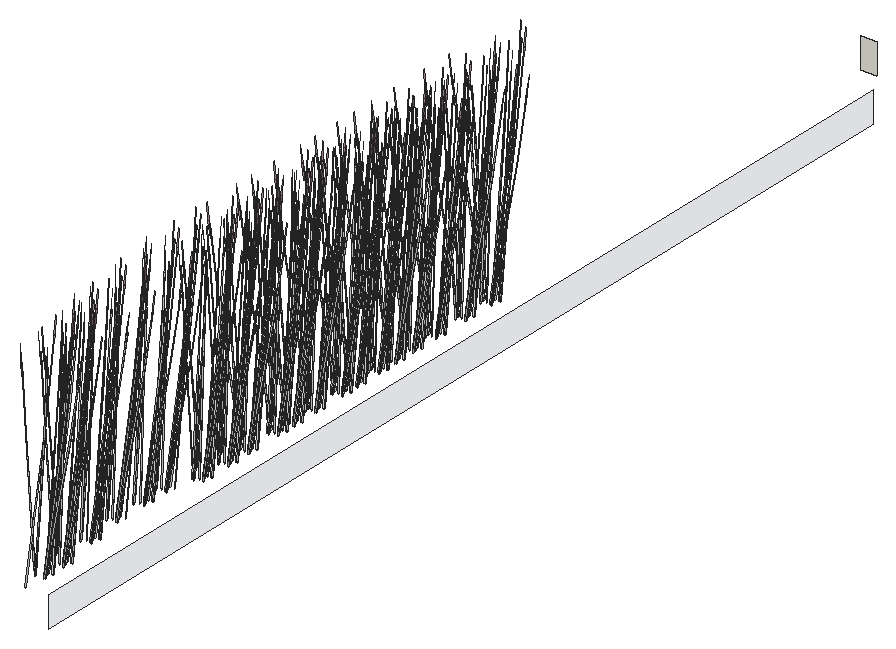
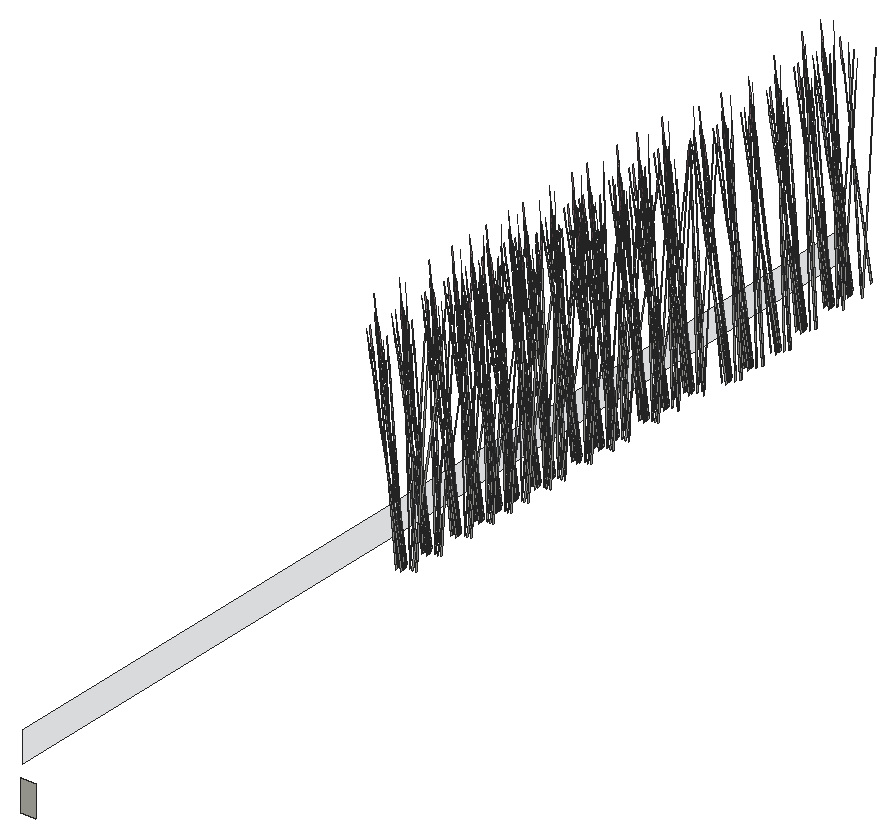
# SketchUp Ruby script. Lengths in inches.
U = 1.inch
M = Sketchup.active_model
def pt(a) = Geom::Point3d.new(a.map { |v| v * U })
def face(e, loops, mat)
  f = e.add_face(loops[0].map { |a| pt(a) })
  loops[1..].each { |l| e.add_face(l.map { |a| pt(a) }).erase! }
  f.material = f.back_material = mat if mat
  f
end
# faces: each face lists its corners as indices into pts; further lists are holes
def faces(e, pts, list, mat = nil) = list.each { |f| face(e, (f[0].is_a?(Array) ? f : [f]).map { |l| l.map { |i| pts[i] } }, mat) }
# xy, xz, yz: faces in a plane at the given z, y or x. An outline is a flat list of corners, or four numbers for a rectangle; further outlines are holes
def ring(l) = l.size == 4 ? [[l[0], l[1]], [l[2], l[1]], [l[2], l[3]], [l[0], l[3]]] : l.each_slice(2).to_a
def flat(e, list, mat, &to3) = list.each { |f| face(e, (f[0].is_a?(Array) ? f : [f]).map { |l| ring(l).map { |u, v| to3.(u, v) } }, mat) }
def xy(e, z, list, mat = nil) = flat(e, list, mat) { |x, y| [x, y, z] }
def xz(e, y, list, mat = nil) = flat(e, list, mat) { |x, z| [x, y, z] }
def yz(e, x, list, mat = nil) = flat(e, list, mat) { |y, z| [x, y, z] }
def lines(e, pts, list) = list.each { |a, b| e.add_line(pt(pts[a]), pt(pts[b])) }
# prism: a flat outline (further loops are holes) pulled along v
def prism(e, loops, v, mat = nil)
  f = face(e, loops, mat); d = Geom::Vector3d.new(v.map { |x| x * U })
  f.pushpull(f.normal.samedirection?(d) ? d.length : -d.length)
end
def box(e, o, s, mat = nil) = prism(e, [[o, [o[0] + s[0], o[1], o[2]], [o[0] + s[0], o[1] + s[1], o[2]], [o[0], o[1] + s[1], o[2]]]], [0, 0, s[2]], mat)
def at(x, y, z, deg = 0) = Geom::Transformation.translation(pt([x, y, z])) * Geom::Transformation.rotation(ORIGIN, Z_AXIS, deg.degrees)
def axes(o, x, y, z) = Geom::Transformation.new([*x, 0, *y, 0, *z, 0, *pt(o).to_a, 1])
def part(name) = M.definitions.add(name)
# library, detail: a bought-in or finely detailed component or shape, given as its bounding box
def library(name, o, s) = part(name).tap { |d| box(d.entities, o, s) }
def detail(e, o, s) = box(e.add_group.entities, o, s)
def put(e, d, t, mat = nil) = e.add_instance(d, t).tap { |i| i.material = mat if mat }
def group(e, t, mat = nil) = e.add_group.tap { |g| g.transformation = t; g.material = mat if mat }.entities
root = M.entities
M.materials.add("D01_Frost_White").color = [238, 238, 227]
M.materials.add("Glass_Basic_01").color = [161, 173, 186]
M.materials["Glass_Basic_01"].alpha = 0.25
M.materials.add("LightPink_Translucent").color = [144, 107, 117]
M.materials["LightPink_Translucent"].alpha = 0.75
c1 = part("blade")
p = [[2.15,0.21,22],[0,0.17,0],[0.09,0.45,0],[2.18,0.31,22],[2.29,0.31,22],[0.38,0.45,0],
  [2.48,0.24,33],[2.49,0.24,33],[2.48,0.22,33]]
faces(c1.entities,p,[[0,1,2,3],[4,5,2,3],[6,3,4,7],[8,0,3,6]])
c2 = part("seeds")
p = [[0.3,-0.1,1.38],[-0.01,-0.03,1.59],[-0.01,-0.03,0.03],[0.14,-0.07,-0.07],[0.29,-0.03,3],[0.15,0.01,3.11]]
faces(c2.entities,p,[[0,1,2,3],[1,0,4,5]],"LightPink_Translucent")
c3 = part("blade with seeds")
put(c3.entities,c1,at(0,0,0))
put(c3.entities,c2,axes([2.4,0.25,30.99],[1.5799,-0.05474,1.17369],[-0.12525,1.92788,0.29478],[-0.07173,-0.02425,1.56792]))
xz(root,586,[[427,150,430,156]],"D01_Frost_White")
yz(root,439,[[373,150,574.02,156]],"Glass_Basic_01")
put(root,c3,axes([428.45,433.25,151.77],[-0.1683,-0.48366,-0.58997],[0.48479,-0.17419,-0.15484],[-0.0186,-0.16378,1.30225]))
put(root,c3,axes([428.45,440.5,151.77],[-0.1683,-0.48366,-0.58997],[0.48479,-0.17419,-0.15484],[-0.0186,-0.16378,1.30225]))
put(root,c3,axes([428.45,444.2,151.77],[-0.1683,-0.48366,-0.58997],[0.48479,-0.17419,-0.15484],[-0.0186,-0.16378,1.30225]))
put(root,c3,axes([428.45,449.62,151.77],[-0.1683,-0.48366,-0.58997],[0.48479,-0.17419,-0.15484],[-0.0186,-0.16378,1.30225]))
put(root,c3,axes([428.45,456.1,151.77],[-0.1683,-0.48366,-0.58997],[0.48479,-0.17419,-0.15484],[-0.0186,-0.16378,1.30225]))
put(root,c3,axes([428.45,459.65,151.77],[-0.1683,-0.48366,-0.58997],[0.48479,-0.17419,-0.15484],[-0.0186,-0.16378,1.30225]))
put(root,c3,axes([428.45,465.05,151.77],[-0.1683,-0.48366,-0.58997],[0.48479,-0.17419,-0.15484],[-0.0186,-0.16378,1.30225]))
put(root,c3,axes([428.45,469.1,151.77],[-0.1683,-0.48366,-0.58997],[0.48479,-0.17419,-0.15484],[-0.0186,-0.16378,1.30225]))
put(root,c3,axes([428.45,473.43,151.77],[-0.1683,-0.48366,-0.58997],[0.48479,-0.17419,-0.15484],[-0.0186,-0.16378,1.30225]))
put(root,c3,axes([428.45,478.97,151.77],[-0.1683,-0.48366,-0.58997],[0.48479,-0.17419,-0.15484],[-0.0186,-0.16378,1.30225]))
put(root,c3,axes([428.45,486.18,151.77],[-0.1683,-0.48366,-0.58997],[0.48479,-0.17419,-0.15484],[-0.0186,-0.16378,1.30225]))
put(root,c3,axes([428.45,492.34,151.77],[-0.1683,-0.48366,-0.58997],[0.48479,-0.17419,-0.15484],[-0.0186,-0.16378,1.30225]))
put(root,c3,axes([427.55,404.96,151.77],[0.15027,0.43184,-0.5847],[-0.43285,0.15553,-0.15346],[0.01661,0.14623,1.29063]))
put(root,c3,axes([428.4,397.25,151.87],[-0.19883,0.425,-0.37796],[-0.41314,-0.20454,0.1819],[0,0.09797,1.2135]))
put(root,c3,axes([428.51,411.5625,151.71],[-0.28606,0.29428,-0.2617],[-0.28606,-0.29428,0.2617],[0,0.09479,1.17405]))
put(root,c3,axes([427.62,416.89,151.77],[0.15027,0.43184,-0.5847],[-0.43285,0.15553,-0.15346],[0.01661,0.14623,1.29063]))
put(root,c3,axes([427.69,411.51,151.77],[0.15027,0.43184,-0.5847],[-0.43285,0.15553,-0.15346],[0.01661,0.14623,1.29063]))
put(root,c3,axes([427.65,383.51,151.71],[0.28606,-0.29428,-0.2617],[0.28606,0.29428,0.2617],[0,-0.09479,1.17405]))
put(root,c3,axes([427.65,388.08,151.71],[0.28606,-0.29428,-0.2617],[0.28606,0.29428,0.2617],[0,-0.09479,1.17405]))
put(root,c3,axes([427.65,422.17,151.71],[0.28606,-0.29428,-0.2617],[0.28606,0.29428,0.2617],[0,-0.09479,1.17405]))
put(root,c3,axes([427.65,428.28,151.71],[0.28606,-0.29428,-0.2617],[0.28606,0.29428,0.2617],[0,-0.09479,1.17405]))
put(root,c3,axes([427.65,433.19,151.71],[0.28606,-0.29428,-0.2617],[0.28606,0.29428,0.2617],[0,-0.09479,1.17405]))
put(root,c3,axes([427.65,440.45,151.71],[0.28606,-0.29428,-0.2617],[0.28606,0.29428,0.2617],[0,-0.09479,1.17405]))
put(root,c3,axes([427.65,444.14,151.71],[0.28606,-0.29428,-0.2617],[0.28606,0.29428,0.2617],[0,-0.09479,1.17405]))
put(root,c3,axes([427.65,449.5625,151.71],[0.28606,-0.29428,-0.2617],[0.28606,0.29428,0.2617],[0,-0.09479,1.17405]))
put(root,c3,axes([427.65,456.04,151.71],[0.28606,-0.29428,-0.2617],[0.28606,0.29428,0.2617],[0,-0.09479,1.17405]))
put(root,c3,axes([427.65,459.59,151.71],[0.28606,-0.29428,-0.2617],[0.28606,0.29428,0.2617],[0,-0.09479,1.17405]))
put(root,c3,axes([427.65,464.99,151.71],[0.28606,-0.29428,-0.2617],[0.28606,0.29428,0.2617],[0,-0.09479,1.17405]))
put(root,c3,axes([427.65,469.05,151.71],[0.28606,-0.29428,-0.2617],[0.28606,0.29428,0.2617],[0,-0.09479,1.17405]))
put(root,c3,axes([427.65,473.37,151.71],[0.28606,-0.29428,-0.2617],[0.28606,0.29428,0.2617],[0,-0.09479,1.17405]))
put(root,c3,axes([427.65,478.91,151.71],[0.28606,-0.29428,-0.2617],[0.28606,0.29428,0.2617],[0,-0.09479,1.17405]))
put(root,c3,axes([427.65,486.12,151.71],[0.28606,-0.29428,-0.2617],[0.28606,0.29428,0.2617],[0,-0.09479,1.17405]))
put(root,c3,axes([427.65,492.29,151.71],[0.28606,-0.29428,-0.2617],[0.28606,0.29428,0.2617],[0,-0.09479,1.17405]))
put(root,c3,axes([426.38,402.86,151.71],[0.38233,0.1167,-0.2617],[-0.09626,0.41098,0.2617],[0.07708,-0.04739,1.17405]))
put(root,c3,axes([426.45,414.79,151.71],[0.38233,0.1167,-0.2617],[-0.09626,0.41098,0.2617],[0.07708,-0.04739,1.17405]))
put(root,c3,axes([426.52,409.41,151.71],[0.38233,0.1167,-0.2617],[-0.09626,0.41098,0.2617],[0.07708,-0.04739,1.17405]))
put(root,c3,axes([428.56,405.02,151.7],[0,0.47166,-0.41945],[-0.45849,0,0],[0,0.10742,1.33059]))
put(root,c3,axes([426.29,402.67,151.7],[0.38354,-0.23583,-0.41945],[0.22925,0.42288,0],[0.08735,-0.05371,1.33059]))
put(root,c3,axes([428.63,416.95,151.7],[0,0.47166,-0.41945],[-0.45849,0,0],[0,0.10742,1.33059]))
put(root,c3,axes([426.36,414.6,151.7],[0.38354,-0.23583,-0.41945],[0.22925,0.42288,0],[0.08735,-0.05371,1.33059]))
put(root,c3,axes([428.7,411.57,151.7],[0,0.47166,-0.41945],[-0.45849,0,0],[0,0.10742,1.33059]))
put(root,c3,axes([426.43,409.22,151.7],[0.38354,-0.23583,-0.41945],[0.22925,0.42288,0],[0.08735,-0.05371,1.33059]))
put(root,c3,axes([429.45,397.43,151.71],[-0.28606,0.29428,-0.2617],[-0.28606,-0.29428,0.2617],[0,0.09479,1.17405]))
put(root,c3,axes([427.28,404.2,151.87],[0.24618,0.39589,-0.37796],[-0.37289,0.27878,0.1819],[0.07967,0.04899,1.2135]))
put(root,c3,axes([428.63,397.38,151.77],[0.15027,0.43184,-0.5847],[-0.43285,0.15553,-0.15346],[0.01661,0.14623,1.29063]))
put(root,c3,axes([427.36,416.14,151.87],[0.24618,0.39589,-0.37796],[-0.37289,0.27878,0.1819],[0.07967,0.04899,1.2135]))
put(root,c3,axes([428.7,388.26,151.87],[0.19883,-0.425,-0.37796],[0.41314,0.20454,0.1819],[0,-0.09797,1.2135]))
put(root,c3,axes([428.7,422.35,151.87],[0.19883,-0.425,-0.37796],[0.41314,0.20454,0.1819],[0,-0.09797,1.2135]))
put(root,c3,axes([428.7,428.46,151.87],[0.19883,-0.425,-0.37796],[0.41314,0.20454,0.1819],[0,-0.09797,1.2135]))
put(root,c3,axes([428.7,433.375,151.87],[0.19883,-0.425,-0.37796],[0.41314,0.20454,0.1819],[0,-0.09797,1.2135]))
put(root,c3,axes([428.7,440.63,151.87],[0.19883,-0.425,-0.37796],[0.41314,0.20454,0.1819],[0,-0.09797,1.2135]))
put(root,c3,axes([428.7,444.32,151.87],[0.19883,-0.425,-0.37796],[0.41314,0.20454,0.1819],[0,-0.09797,1.2135]))
put(root,c3,axes([428.7,449.74,151.87],[0.19883,-0.425,-0.37796],[0.41314,0.20454,0.1819],[0,-0.09797,1.2135]))
put(root,c3,axes([428.7,456.23,151.87],[0.19883,-0.425,-0.37796],[0.41314,0.20454,0.1819],[0,-0.09797,1.2135]))
put(root,c3,axes([428.7,459.77,151.87],[0.19883,-0.425,-0.37796],[0.41314,0.20454,0.1819],[0,-0.09797,1.2135]))
put(root,c3,axes([428.7,465.18,151.87],[0.19883,-0.425,-0.37796],[0.41314,0.20454,0.1819],[0,-0.09797,1.2135]))
put(root,c3,axes([428.7,469.23,151.87],[0.19883,-0.425,-0.37796],[0.41314,0.20454,0.1819],[0,-0.09797,1.2135]))
put(root,c3,axes([428.7,473.55,151.87],[0.19883,-0.425,-0.37796],[0.41314,0.20454,0.1819],[0,-0.09797,1.2135]))
put(root,c3,axes([428.7,479.09,151.87],[0.19883,-0.425,-0.37796],[0.41314,0.20454,0.1819],[0,-0.09797,1.2135]))
put(root,c3,axes([428.7,486.3,151.87],[0.19883,-0.425,-0.37796],[0.41314,0.20454,0.1819],[0,-0.09797,1.2135]))
put(root,c3,axes([428.7,492.47,151.87],[0.19883,-0.425,-0.37796],[0.41314,0.20454,0.1819],[0,-0.09797,1.2135]))
put(root,c3,axes([427.43,410.75,151.87],[0.24618,0.39589,-0.37796],[-0.37289,0.27878,0.1819],[0.07967,0.04899,1.2135]))
put(root,c3,axes([426.74,403.64,151.74],[0.27603,-0.35451,-0.52676],[0.34289,0.32147,-0.13825],[0.11061,-0.08844,1.16273]))
put(root,c3,axes([426.82,415.57,151.74],[0.27603,-0.35451,-0.52676],[0.34289,0.32147,-0.13825],[0.11061,-0.08844,1.16273]))
put(root,c3,axes([426.89,410.19,151.74],[0.27603,-0.35451,-0.52676],[0.34289,0.32147,-0.13825],[0.11061,-0.08844,1.16273]))
put(root,c3,axes([429.75,384.26,151.87],[-0.19883,0.425,-0.37796],[-0.41314,-0.20454,0.1819],[0,0.09797,1.2135]))
put(root,c3,axes([429.75,388.83,151.87],[-0.19883,0.425,-0.37796],[-0.41314,-0.20454,0.1819],[0,0.09797,1.2135]))
put(root,c3,axes([429.75,422.92,151.87],[-0.19883,0.425,-0.37796],[-0.41314,-0.20454,0.1819],[0,0.09797,1.2135]))
put(root,c3,axes([429.75,429.03,151.87],[-0.19883,0.425,-0.37796],[-0.41314,-0.20454,0.1819],[0,0.09797,1.2135]))
put(root,c3,axes([429.75,433.94,151.87],[-0.19883,0.425,-0.37796],[-0.41314,-0.20454,0.1819],[0,0.09797,1.2135]))
put(root,c3,axes([429.75,441.2,151.87],[-0.19883,0.425,-0.37796],[-0.41314,-0.20454,0.1819],[0,0.09797,1.2135]))
put(root,c3,axes([429.75,444.89,151.87],[-0.19883,0.425,-0.37796],[-0.41314,-0.20454,0.1819],[0,0.09797,1.2135]))
put(root,c3,axes([429.75,450.3125,151.87],[-0.19883,0.425,-0.37796],[-0.41314,-0.20454,0.1819],[0,0.09797,1.2135]))
put(root,c3,axes([429.75,456.79,151.87],[-0.19883,0.425,-0.37796],[-0.41314,-0.20454,0.1819],[0,0.09797,1.2135]))
put(root,c3,axes([429.75,460.34,151.87],[-0.19883,0.425,-0.37796],[-0.41314,-0.20454,0.1819],[0,0.09797,1.2135]))
put(root,c3,axes([429.75,465.74,151.87],[-0.19883,0.425,-0.37796],[-0.41314,-0.20454,0.1819],[0,0.09797,1.2135]))
put(root,c3,axes([429.75,469.8,151.87],[-0.19883,0.425,-0.37796],[-0.41314,-0.20454,0.1819],[0,0.09797,1.2135]))
put(root,c3,axes([429.75,474.12,151.87],[-0.19883,0.425,-0.37796],[-0.41314,-0.20454,0.1819],[0,0.09797,1.2135]))
put(root,c3,axes([429.75,479.66,151.87],[-0.19883,0.425,-0.37796],[-0.41314,-0.20454,0.1819],[0,0.09797,1.2135]))
put(root,c3,axes([429.75,486.87,151.87],[-0.19883,0.425,-0.37796],[-0.41314,-0.20454,0.1819],[0,0.09797,1.2135]))
put(root,c3,axes([429.75,493.04,151.87],[-0.19883,0.425,-0.37796],[-0.41314,-0.20454,0.1819],[0,0.09797,1.2135]))
put(root,c3,axes([427.46,395.28,151.71],[0.38233,0.1167,-0.2617],[-0.09626,0.41098,0.2617],[0.07708,-0.04739,1.17405]))
put(root,c3,axes([427.95,403.33,151.71],[0.09626,0.41098,-0.2617],[-0.38233,0.1167,0.2617],[0.07708,0.04739,1.17405]))
put(root,c3,axes([428.03,415.26,151.71],[0.09626,0.41098,-0.2617],[-0.38233,0.1167,0.2617],[0.07708,0.04739,1.17405]))
put(root,c3,axes([429.64,397.45,151.7],[0,0.47166,-0.41945],[-0.45849,0,0],[0,0.10742,1.33059]))
put(root,c3,axes([428.1,409.875,151.71],[0.09626,0.41098,-0.2617],[-0.38233,0.1167,0.2617],[0.07708,0.04739,1.17405]))
put(root,c3,axes([427.375,395.1,151.7],[0.38354,-0.23583,-0.41945],[0.22925,0.42288,0],[0.08735,-0.05371,1.33059]))
put(root,c3,axes([428.37,396.625,151.87],[0.24618,0.39589,-0.37796],[-0.37289,0.27878,0.1819],[0.07967,0.04899,1.2135]))
put(root,c3,axes([428.0625,403.15,151.7],[0.38354,0.23583,-0.41945],[-0.22925,0.42288,0],[0.08735,0.05371,1.33059]))
put(root,c3,axes([428.14,415.08,151.7],[0.38354,0.23583,-0.41945],[-0.22925,0.42288,0],[0.08735,0.05371,1.33059]))
put(root,c3,axes([428.21,409.7,151.7],[0.38354,0.23583,-0.41945],[-0.22925,0.42288,0],[0.08735,0.05371,1.33059]))
put(root,c3,axes([427.83,396.0625,151.74],[0.27603,-0.35451,-0.52676],[0.34289,0.32147,-0.13825],[0.11061,-0.08844,1.16273]))
put(root,c3,axes([430.8,384.4375,151.71],[-0.28606,0.29428,-0.2617],[-0.28606,-0.29428,0.2617],[0,0.09479,1.17405]))
put(root,c3,axes([430.8,389.01,151.71],[-0.28606,0.29428,-0.2617],[-0.28606,-0.29428,0.2617],[0,0.09479,1.17405]))
put(root,c3,axes([430.8,423.1,151.71],[-0.28606,0.29428,-0.2617],[-0.28606,-0.29428,0.2617],[0,0.09479,1.17405]))
put(root,c3,axes([430.8,429.21,151.71],[-0.28606,0.29428,-0.2617],[-0.28606,-0.29428,0.2617],[0,0.09479,1.17405]))
put(root,c3,axes([430.8,434.125,151.71],[-0.28606,0.29428,-0.2617],[-0.28606,-0.29428,0.2617],[0,0.09479,1.17405]))
put(root,c3,axes([430.8,441.38,151.71],[-0.28606,0.29428,-0.2617],[-0.28606,-0.29428,0.2617],[0,0.09479,1.17405]))
put(root,c3,axes([430.8,445.07,151.71],[-0.28606,0.29428,-0.2617],[-0.28606,-0.29428,0.2617],[0,0.09479,1.17405]))
put(root,c3,axes([430.8,450.49,151.71],[-0.28606,0.29428,-0.2617],[-0.28606,-0.29428,0.2617],[0,0.09479,1.17405]))
put(root,c3,axes([430.8,456.98,151.71],[-0.28606,0.29428,-0.2617],[-0.28606,-0.29428,0.2617],[0,0.09479,1.17405]))
put(root,c3,axes([430.8,460.52,151.71],[-0.28606,0.29428,-0.2617],[-0.28606,-0.29428,0.2617],[0,0.09479,1.17405]))
put(root,c3,axes([430.8,465.93,151.71],[-0.28606,0.29428,-0.2617],[-0.28606,-0.29428,0.2617],[0,0.09479,1.17405]))
put(root,c3,axes([430.8,469.98,151.71],[-0.28606,0.29428,-0.2617],[-0.28606,-0.29428,0.2617],[0,0.09479,1.17405]))
put(root,c3,axes([430.8,474.31,151.71],[-0.28606,0.29428,-0.2617],[-0.28606,-0.29428,0.2617],[0,0.09479,1.17405]))
put(root,c3,axes([430.8,479.84,151.71],[-0.28606,0.29428,-0.2617],[-0.28606,-0.29428,0.2617],[0,0.09479,1.17405]))
put(root,c3,axes([430.8,487.05,151.71],[-0.28606,0.29428,-0.2617],[-0.28606,-0.29428,0.2617],[0,0.09479,1.17405]))
put(root,c3,axes([430.8,493.22,151.71],[-0.28606,0.29428,-0.2617],[-0.28606,-0.29428,0.2617],[0,0.09479,1.17405]))
put(root,c3,axes([427.5,404.05,151.74],[0.42629,0.07733,-0.52676],[-0.08996,0.47699,-0.13825],[0.12722,0.0578,1.16273]))
put(root,c3,axes([429.99,378.64,151.77],[0.15027,0.43184,-0.5847],[-0.43285,0.15553,-0.15346],[0.01661,0.14623,1.29063]))
put(root,c3,axes([429.99,384.38,151.77],[0.15027,0.43184,-0.5847],[-0.43285,0.15553,-0.15346],[0.01661,0.14623,1.29063]))
put(root,c3,axes([429.99,388.96,151.77],[0.15027,0.43184,-0.5847],[-0.43285,0.15553,-0.15346],[0.01661,0.14623,1.29063]))
put(root,c3,axes([429.99,423.05,151.77],[0.15027,0.43184,-0.5847],[-0.43285,0.15553,-0.15346],[0.01661,0.14623,1.29063]))
put(root,c3,axes([429.99,429.16,151.77],[0.15027,0.43184,-0.5847],[-0.43285,0.15553,-0.15346],[0.01661,0.14623,1.29063]))
put(root,c3,axes([429.99,434.07,151.77],[0.15027,0.43184,-0.5847],[-0.43285,0.15553,-0.15346],[0.01661,0.14623,1.29063]))
put(root,c3,axes([429.99,441.33,151.77],[0.15027,0.43184,-0.5847],[-0.43285,0.15553,-0.15346],[0.01661,0.14623,1.29063]))
put(root,c3,axes([429.99,445.02,151.77],[0.15027,0.43184,-0.5847],[-0.43285,0.15553,-0.15346],[0.01661,0.14623,1.29063]))
put(root,c3,axes([429.99,450.44,151.77],[0.15027,0.43184,-0.5847],[-0.43285,0.15553,-0.15346],[0.01661,0.14623,1.29063]))
put(root,c3,axes([429.99,456.92,151.77],[0.15027,0.43184,-0.5847],[-0.43285,0.15553,-0.15346],[0.01661,0.14623,1.29063]))
put(root,c3,axes([429.99,460.47,151.77],[0.15027,0.43184,-0.5847],[-0.43285,0.15553,-0.15346],[0.01661,0.14623,1.29063]))
put(root,c3,axes([429.99,465.87,151.77],[0.15027,0.43184,-0.5847],[-0.43285,0.15553,-0.15346],[0.01661,0.14623,1.29063]))
put(root,c3,axes([429.99,469.93,151.77],[0.15027,0.43184,-0.5847],[-0.43285,0.15553,-0.15346],[0.01661,0.14623,1.29063]))
put(root,c3,axes([429.99,474.25,151.77],[0.15027,0.43184,-0.5847],[-0.43285,0.15553,-0.15346],[0.01661,0.14623,1.29063]))
put(root,c3,axes([429.99,479.79,151.77],[0.15027,0.43184,-0.5847],[-0.43285,0.15553,-0.15346],[0.01661,0.14623,1.29063]))
put(root,c3,axes([429.99,487,151.77],[0.15027,0.43184,-0.5847],[-0.43285,0.15553,-0.15346],[0.01661,0.14623,1.29063]))
put(root,c3,axes([429.99,493.17,151.77],[0.15027,0.43184,-0.5847],[-0.43285,0.15553,-0.15346],[0.01661,0.14623,1.29063]))
put(root,c3,axes([427.58,415.98,151.74],[0.42629,0.07733,-0.52676],[-0.08996,0.47699,-0.13825],[0.12722,0.0578,1.16273]))
put(root,c3,axes([429.04,395.75,151.71],[0.09626,0.41098,-0.2617],[-0.38233,0.1167,0.2617],[0.07708,0.04739,1.17405]))
put(root,c3,axes([427.65,410.6,151.74],[0.42629,0.07733,-0.52676],[-0.08996,0.47699,-0.13825],[0.12722,0.0578,1.16273]))
put(root,c3,axes([428.82,382.29,151.71],[0.38233,0.1167,-0.2617],[-0.09626,0.41098,0.2617],[0.07708,-0.04739,1.17405]))
put(root,c3,axes([428.82,386.86,151.71],[0.38233,0.1167,-0.2617],[-0.09626,0.41098,0.2617],[0.07708,-0.04739,1.17405]))
put(root,c3,axes([428.82,420.95,151.71],[0.38233,0.1167,-0.2617],[-0.09626,0.41098,0.2617],[0.07708,-0.04739,1.17405]))
put(root,c3,axes([428.82,427.06,151.71],[0.38233,0.1167,-0.2617],[-0.09626,0.41098,0.2617],[0.07708,-0.04739,1.17405]))
put(root,c3,axes([428.82,431.97,151.71],[0.38233,0.1167,-0.2617],[-0.09626,0.41098,0.2617],[0.07708,-0.04739,1.17405]))
put(root,c3,axes([428.82,439.23,151.71],[0.38233,0.1167,-0.2617],[-0.09626,0.41098,0.2617],[0.07708,-0.04739,1.17405]))
put(root,c3,axes([428.82,442.92,151.71],[0.38233,0.1167,-0.2617],[-0.09626,0.41098,0.2617],[0.07708,-0.04739,1.17405]))
put(root,c3,axes([428.82,448.34,151.71],[0.38233,0.1167,-0.2617],[-0.09626,0.41098,0.2617],[0.07708,-0.04739,1.17405]))
put(root,c3,axes([428.82,454.82,151.71],[0.38233,0.1167,-0.2617],[-0.09626,0.41098,0.2617],[0.07708,-0.04739,1.17405]))
put(root,c3,axes([428.82,458.37,151.71],[0.38233,0.1167,-0.2617],[-0.09626,0.41098,0.2617],[0.07708,-0.04739,1.17405]))
put(root,c3,axes([428.82,463.77,151.71],[0.38233,0.1167,-0.2617],[-0.09626,0.41098,0.2617],[0.07708,-0.04739,1.17405]))
put(root,c3,axes([428.82,467.83,151.71],[0.38233,0.1167,-0.2617],[-0.09626,0.41098,0.2617],[0.07708,-0.04739,1.17405]))
put(root,c3,axes([428.82,472.15,151.71],[0.38233,0.1167,-0.2617],[-0.09626,0.41098,0.2617],[0.07708,-0.04739,1.17405]))
put(root,c3,axes([428.82,477.6875,151.71],[0.38233,0.1167,-0.2617],[-0.09626,0.41098,0.2617],[0.07708,-0.04739,1.17405]))
put(root,c3,axes([428.82,484.9,151.71],[0.38233,0.1167,-0.2617],[-0.09626,0.41098,0.2617],[0.07708,-0.04739,1.17405]))
put(root,c3,axes([428.82,491.07,151.71],[0.38233,0.1167,-0.2617],[-0.09626,0.41098,0.2617],[0.07708,-0.04739,1.17405]))
put(root,c3,axes([431,384.45,151.7],[0,0.47166,-0.41945],[-0.45849,0,0],[0,0.10742,1.33059]))
put(root,c3,axes([431,389.02,151.7],[0,0.47166,-0.41945],[-0.45849,0,0],[0,0.10742,1.33059]))
put(root,c3,axes([431,423.11,151.7],[0,0.47166,-0.41945],[-0.45849,0,0],[0,0.10742,1.33059]))
put(root,c3,axes([431,429.22,151.7],[0,0.47166,-0.41945],[-0.45849,0,0],[0,0.10742,1.33059]))
put(root,c3,axes([431,434.14,151.7],[0,0.47166,-0.41945],[-0.45849,0,0],[0,0.10742,1.33059]))
put(root,c3,axes([431,441.39,151.7],[0,0.47166,-0.41945],[-0.45849,0,0],[0,0.10742,1.33059]))
put(root,c3,axes([431,445.08,151.7],[0,0.47166,-0.41945],[-0.45849,0,0],[0,0.10742,1.33059]))
put(root,c3,axes([431,450.5,151.7],[0,0.47166,-0.41945],[-0.45849,0,0],[0,0.10742,1.33059]))
put(root,c3,axes([431,456.99,151.7],[0,0.47166,-0.41945],[-0.45849,0,0],[0,0.10742,1.33059]))
put(root,c3,axes([431,460.53,151.7],[0,0.47166,-0.41945],[-0.45849,0,0],[0,0.10742,1.33059]))
put(root,c3,axes([431,465.9375,151.7],[0,0.47166,-0.41945],[-0.45849,0,0],[0,0.10742,1.33059]))
put(root,c3,axes([431,469.99,151.7],[0,0.47166,-0.41945],[-0.45849,0,0],[0,0.10742,1.33059]))
put(root,c3,axes([431,474.32,151.7],[0,0.47166,-0.41945],[-0.45849,0,0],[0,0.10742,1.33059]))
put(root,c3,axes([431,479.85,151.7],[0,0.47166,-0.41945],[-0.45849,0,0],[0,0.10742,1.33059]))
put(root,c3,axes([431,487.06,151.7],[0,0.47166,-0.41945],[-0.45849,0,0],[0,0.10742,1.33059]))
put(root,c3,axes([431,493.23,151.7],[0,0.47166,-0.41945],[-0.45849,0,0],[0,0.10742,1.33059]))
put(root,c3,axes([428.73,386.67,151.7],[0.38354,-0.23583,-0.41945],[0.22925,0.42288,0],[0.08735,-0.05371,1.33059]))
put(root,c3,axes([428.73,420.76,151.7],[0.38354,-0.23583,-0.41945],[0.22925,0.42288,0],[0.08735,-0.05371,1.33059]))
put(root,c3,axes([428.73,426.87,151.7],[0.38354,-0.23583,-0.41945],[0.22925,0.42288,0],[0.08735,-0.05371,1.33059]))
put(root,c3,axes([428.73,431.79,151.7],[0.38354,-0.23583,-0.41945],[0.22925,0.42288,0],[0.08735,-0.05371,1.33059]))
put(root,c3,axes([428.73,439.04,151.7],[0.38354,-0.23583,-0.41945],[0.22925,0.42288,0],[0.08735,-0.05371,1.33059]))
put(root,c3,axes([428.73,442.73,151.7],[0.38354,-0.23583,-0.41945],[0.22925,0.42288,0],[0.08735,-0.05371,1.33059]))
put(root,c3,axes([428.73,448.15,151.7],[0.38354,-0.23583,-0.41945],[0.22925,0.42288,0],[0.08735,-0.05371,1.33059]))
put(root,c3,axes([428.73,454.64,151.7],[0.38354,-0.23583,-0.41945],[0.22925,0.42288,0],[0.08735,-0.05371,1.33059]))
put(root,c3,axes([428.73,458.18,151.7],[0.38354,-0.23583,-0.41945],[0.22925,0.42288,0],[0.08735,-0.05371,1.33059]))
put(root,c3,axes([428.73,463.59,151.7],[0.38354,-0.23583,-0.41945],[0.22925,0.42288,0],[0.08735,-0.05371,1.33059]))
put(root,c3,axes([428.73,467.64,151.7],[0.38354,-0.23583,-0.41945],[0.22925,0.42288,0],[0.08735,-0.05371,1.33059]))
put(root,c3,axes([428.73,471.97,151.7],[0.38354,-0.23583,-0.41945],[0.22925,0.42288,0],[0.08735,-0.05371,1.33059]))
put(root,c3,axes([428.73,477.5,151.7],[0.38354,-0.23583,-0.41945],[0.22925,0.42288,0],[0.08735,-0.05371,1.33059]))
put(root,c3,axes([428.73,484.71,151.7],[0.38354,-0.23583,-0.41945],[0.22925,0.42288,0],[0.08735,-0.05371,1.33059]))
put(root,c3,axes([428.73,490.88,151.7],[0.38354,-0.23583,-0.41945],[0.22925,0.42288,0],[0.08735,-0.05371,1.33059]))
put(root,c3,axes([429.15,395.57,151.7],[0.38354,0.23583,-0.41945],[-0.22925,0.42288,0],[0.08735,0.05371,1.33059]))
put(root,c3,axes([429.72,383.63,151.87],[0.24618,0.39589,-0.37796],[-0.37289,0.27878,0.1819],[0.07967,0.04899,1.2135]))
put(root,c3,axes([429.72,388.2,151.87],[0.24618,0.39589,-0.37796],[-0.37289,0.27878,0.1819],[0.07967,0.04899,1.2135]))
put(root,c3,axes([429.72,422.29,151.87],[0.24618,0.39589,-0.37796],[-0.37289,0.27878,0.1819],[0.07967,0.04899,1.2135]))
put(root,c3,axes([429.72,428.4,151.87],[0.24618,0.39589,-0.37796],[-0.37289,0.27878,0.1819],[0.07967,0.04899,1.2135]))
put(root,c3,axes([429.72,433.32,151.87],[0.24618,0.39589,-0.37796],[-0.37289,0.27878,0.1819],[0.07967,0.04899,1.2135]))
put(root,c3,axes([429.72,440.57,151.87],[0.24618,0.39589,-0.37796],[-0.37289,0.27878,0.1819],[0.07967,0.04899,1.2135]))
put(root,c3,axes([429.72,444.26,151.87],[0.24618,0.39589,-0.37796],[-0.37289,0.27878,0.1819],[0.07967,0.04899,1.2135]))
put(root,c3,axes([429.72,449.6875,151.87],[0.24618,0.39589,-0.37796],[-0.37289,0.27878,0.1819],[0.07967,0.04899,1.2135]))
put(root,c3,axes([429.72,456.17,151.87],[0.24618,0.39589,-0.37796],[-0.37289,0.27878,0.1819],[0.07967,0.04899,1.2135]))
put(root,c3,axes([429.72,459.72,151.87],[0.24618,0.39589,-0.37796],[-0.37289,0.27878,0.1819],[0.07967,0.04899,1.2135]))
put(root,c3,axes([429.72,465.12,151.87],[0.24618,0.39589,-0.37796],[-0.37289,0.27878,0.1819],[0.07967,0.04899,1.2135]))
put(root,c3,axes([429.72,469.17,151.87],[0.24618,0.39589,-0.37796],[-0.37289,0.27878,0.1819],[0.07967,0.04899,1.2135]))
put(root,c3,axes([429.72,473.5,151.87],[0.24618,0.39589,-0.37796],[-0.37289,0.27878,0.1819],[0.07967,0.04899,1.2135]))
put(root,c3,axes([429.72,479.03,151.87],[0.24618,0.39589,-0.37796],[-0.37289,0.27878,0.1819],[0.07967,0.04899,1.2135]))
put(root,c3,axes([429.72,486.25,151.87],[0.24618,0.39589,-0.37796],[-0.37289,0.27878,0.1819],[0.07967,0.04899,1.2135]))
put(root,c3,axes([429.72,492.41,151.87],[0.24618,0.39589,-0.37796],[-0.37289,0.27878,0.1819],[0.07967,0.04899,1.2135]))
put(root,c3,axes([428.59,396.48,151.74],[0.42629,0.07733,-0.52676],[-0.08996,0.47699,-0.13825],[0.12722,0.0578,1.16273]))
put(root,c3,axes([429.19,387.64,151.74],[0.27603,-0.35451,-0.52676],[0.34289,0.32147,-0.13825],[0.11061,-0.08844,1.16273]))
put(root,c3,axes([429.19,421.73,151.74],[0.27603,-0.35451,-0.52676],[0.34289,0.32147,-0.13825],[0.11061,-0.08844,1.16273]))
put(root,c3,axes([429.19,427.84,151.74],[0.27603,-0.35451,-0.52676],[0.34289,0.32147,-0.13825],[0.11061,-0.08844,1.16273]))
put(root,c3,axes([429.19,432.75,151.74],[0.27603,-0.35451,-0.52676],[0.34289,0.32147,-0.13825],[0.11061,-0.08844,1.16273]))
put(root,c3,axes([429.19,440.01,151.74],[0.27603,-0.35451,-0.52676],[0.34289,0.32147,-0.13825],[0.11061,-0.08844,1.16273]))
put(root,c3,axes([429.19,443.7,151.74],[0.27603,-0.35451,-0.52676],[0.34289,0.32147,-0.13825],[0.11061,-0.08844,1.16273]))
put(root,c3,axes([429.19,449.12,151.74],[0.27603,-0.35451,-0.52676],[0.34289,0.32147,-0.13825],[0.11061,-0.08844,1.16273]))
put(root,c3,axes([429.19,455.6,151.74],[0.27603,-0.35451,-0.52676],[0.34289,0.32147,-0.13825],[0.11061,-0.08844,1.16273]))
put(root,c3,axes([429.19,459.15,151.74],[0.27603,-0.35451,-0.52676],[0.34289,0.32147,-0.13825],[0.11061,-0.08844,1.16273]))
put(root,c3,axes([429.19,464.55,151.74],[0.27603,-0.35451,-0.52676],[0.34289,0.32147,-0.13825],[0.11061,-0.08844,1.16273]))
put(root,c3,axes([429.19,468.61,151.74],[0.27603,-0.35451,-0.52676],[0.34289,0.32147,-0.13825],[0.11061,-0.08844,1.16273]))
put(root,c3,axes([429.19,472.93,151.74],[0.27603,-0.35451,-0.52676],[0.34289,0.32147,-0.13825],[0.11061,-0.08844,1.16273]))
put(root,c3,axes([429.19,478.47,151.74],[0.27603,-0.35451,-0.52676],[0.34289,0.32147,-0.13825],[0.11061,-0.08844,1.16273]))
put(root,c3,axes([429.19,485.68,151.74],[0.27603,-0.35451,-0.52676],[0.34289,0.32147,-0.13825],[0.11061,-0.08844,1.16273]))
put(root,c3,axes([429.19,491.85,151.74],[0.27603,-0.35451,-0.52676],[0.34289,0.32147,-0.13825],[0.11061,-0.08844,1.16273]))
put(root,c3,axes([430.4,382.75,151.71],[0.09626,0.41098,-0.2617],[-0.38233,0.1167,0.2617],[0.07708,0.04739,1.17405]))
put(root,c3,axes([430.4,387.32,151.71],[0.09626,0.41098,-0.2617],[-0.38233,0.1167,0.2617],[0.07708,0.04739,1.17405]))
put(root,c3,axes([430.4,421.41,151.71],[0.09626,0.41098,-0.2617],[-0.38233,0.1167,0.2617],[0.07708,0.04739,1.17405]))
put(root,c3,axes([430.4,427.53,151.71],[0.09626,0.41098,-0.2617],[-0.38233,0.1167,0.2617],[0.07708,0.04739,1.17405]))
put(root,c3,axes([430.4,432.4375,151.71],[0.09626,0.41098,-0.2617],[-0.38233,0.1167,0.2617],[0.07708,0.04739,1.17405]))
put(root,c3,axes([430.4,439.69,151.71],[0.09626,0.41098,-0.2617],[-0.38233,0.1167,0.2617],[0.07708,0.04739,1.17405]))
put(root,c3,axes([430.4,443.39,151.71],[0.09626,0.41098,-0.2617],[-0.38233,0.1167,0.2617],[0.07708,0.04739,1.17405]))
put(root,c3,axes([430.4,448.81,151.71],[0.09626,0.41098,-0.2617],[-0.38233,0.1167,0.2617],[0.07708,0.04739,1.17405]))
put(root,c3,axes([430.4,455.29,151.71],[0.09626,0.41098,-0.2617],[-0.38233,0.1167,0.2617],[0.07708,0.04739,1.17405]))
put(root,c3,axes([430.4,458.84,151.71],[0.09626,0.41098,-0.2617],[-0.38233,0.1167,0.2617],[0.07708,0.04739,1.17405]))
put(root,c3,axes([430.4,464.24,151.71],[0.09626,0.41098,-0.2617],[-0.38233,0.1167,0.2617],[0.07708,0.04739,1.17405]))
put(root,c3,axes([430.4,468.29,151.71],[0.09626,0.41098,-0.2617],[-0.38233,0.1167,0.2617],[0.07708,0.04739,1.17405]))
put(root,c3,axes([430.4,472.62,151.71],[0.09626,0.41098,-0.2617],[-0.38233,0.1167,0.2617],[0.07708,0.04739,1.17405]))
put(root,c3,axes([430.4,478.15,151.71],[0.09626,0.41098,-0.2617],[-0.38233,0.1167,0.2617],[0.07708,0.04739,1.17405]))
put(root,c3,axes([430.4,485.37,151.71],[0.09626,0.41098,-0.2617],[-0.38233,0.1167,0.2617],[0.07708,0.04739,1.17405]))
put(root,c3,axes([430.4,491.53,151.71],[0.09626,0.41098,-0.2617],[-0.38233,0.1167,0.2617],[0.07708,0.04739,1.17405]))
put(root,c3,axes([430.5,382.58,151.7],[0.38354,0.23583,-0.41945],[-0.22925,0.42288,0],[0.08735,0.05371,1.33059]))
put(root,c3,axes([430.5,387.15,151.7],[0.38354,0.23583,-0.41945],[-0.22925,0.42288,0],[0.08735,0.05371,1.33059]))
put(root,c3,axes([430.5,421.24,151.7],[0.38354,0.23583,-0.41945],[-0.22925,0.42288,0],[0.08735,0.05371,1.33059]))
put(root,c3,axes([430.5,427.35,151.7],[0.38354,0.23583,-0.41945],[-0.22925,0.42288,0],[0.08735,0.05371,1.33059]))
put(root,c3,axes([430.5,432.26,151.7],[0.38354,0.23583,-0.41945],[-0.22925,0.42288,0],[0.08735,0.05371,1.33059]))
put(root,c3,axes([430.5,439.52,151.7],[0.38354,0.23583,-0.41945],[-0.22925,0.42288,0],[0.08735,0.05371,1.33059]))
put(root,c3,axes([430.5,443.21,151.7],[0.38354,0.23583,-0.41945],[-0.22925,0.42288,0],[0.08735,0.05371,1.33059]))
put(root,c3,axes([430.5,448.63,151.7],[0.38354,0.23583,-0.41945],[-0.22925,0.42288,0],[0.08735,0.05371,1.33059]))
put(root,c3,axes([430.5,455.11,151.7],[0.38354,0.23583,-0.41945],[-0.22925,0.42288,0],[0.08735,0.05371,1.33059]))
put(root,c3,axes([430.5,458.66,151.7],[0.38354,0.23583,-0.41945],[-0.22925,0.42288,0],[0.08735,0.05371,1.33059]))
put(root,c3,axes([430.5,464.0625,151.7],[0.38354,0.23583,-0.41945],[-0.22925,0.42288,0],[0.08735,0.05371,1.33059]))
put(root,c3,axes([430.5,468.12,151.7],[0.38354,0.23583,-0.41945],[-0.22925,0.42288,0],[0.08735,0.05371,1.33059]))
put(root,c3,axes([430.5,472.44,151.7],[0.38354,0.23583,-0.41945],[-0.22925,0.42288,0],[0.08735,0.05371,1.33059]))
put(root,c3,axes([430.5,477.98,151.7],[0.38354,0.23583,-0.41945],[-0.22925,0.42288,0],[0.08735,0.05371,1.33059]))
put(root,c3,axes([430.5,485.19,151.7],[0.38354,0.23583,-0.41945],[-0.22925,0.42288,0],[0.08735,0.05371,1.33059]))
put(root,c3,axes([430.5,491.36,151.7],[0.38354,0.23583,-0.41945],[-0.22925,0.42288,0],[0.08735,0.05371,1.33059]))
put(root,c3,axes([429.94,383.48,151.74],[0.42629,0.07733,-0.52676],[-0.08996,0.47699,-0.13825],[0.12722,0.0578,1.16273]))
put(root,c3,axes([429.94,388.05,151.74],[0.42629,0.07733,-0.52676],[-0.08996,0.47699,-0.13825],[0.12722,0.0578,1.16273]))
put(root,c3,axes([429.94,422.14,151.74],[0.42629,0.07733,-0.52676],[-0.08996,0.47699,-0.13825],[0.12722,0.0578,1.16273]))
put(root,c3,axes([429.94,428.25,151.74],[0.42629,0.07733,-0.52676],[-0.08996,0.47699,-0.13825],[0.12722,0.0578,1.16273]))
put(root,c3,axes([429.94,433.17,151.74],[0.42629,0.07733,-0.52676],[-0.08996,0.47699,-0.13825],[0.12722,0.0578,1.16273]))
put(root,c3,axes([429.94,440.42,151.74],[0.42629,0.07733,-0.52676],[-0.08996,0.47699,-0.13825],[0.12722,0.0578,1.16273]))
put(root,c3,axes([429.94,444.11,151.74],[0.42629,0.07733,-0.52676],[-0.08996,0.47699,-0.13825],[0.12722,0.0578,1.16273]))
put(root,c3,axes([429.94,449.53,151.74],[0.42629,0.07733,-0.52676],[-0.08996,0.47699,-0.13825],[0.12722,0.0578,1.16273]))
put(root,c3,axes([429.94,456.02,151.74],[0.42629,0.07733,-0.52676],[-0.08996,0.47699,-0.13825],[0.12722,0.0578,1.16273]))
put(root,c3,axes([429.94,459.5625,151.74],[0.42629,0.07733,-0.52676],[-0.08996,0.47699,-0.13825],[0.12722,0.0578,1.16273]))
put(root,c3,axes([429.94,464.97,151.74],[0.42629,0.07733,-0.52676],[-0.08996,0.47699,-0.13825],[0.12722,0.0578,1.16273]))
put(root,c3,axes([429.94,469.02,151.74],[0.42629,0.07733,-0.52676],[-0.08996,0.47699,-0.13825],[0.12722,0.0578,1.16273]))
put(root,c3,axes([429.94,473.35,151.74],[0.42629,0.07733,-0.52676],[-0.08996,0.47699,-0.13825],[0.12722,0.0578,1.16273]))
put(root,c3,axes([429.94,478.88,151.74],[0.42629,0.07733,-0.52676],[-0.08996,0.47699,-0.13825],[0.12722,0.0578,1.16273]))
put(root,c3,axes([429.94,486.09,151.74],[0.42629,0.07733,-0.52676],[-0.08996,0.47699,-0.13825],[0.12722,0.0578,1.16273]))
put(root,c3,axes([429.94,492.26,151.74],[0.42629,0.07733,-0.52676],[-0.08996,0.47699,-0.13825],[0.12722,0.0578,1.16273]))
